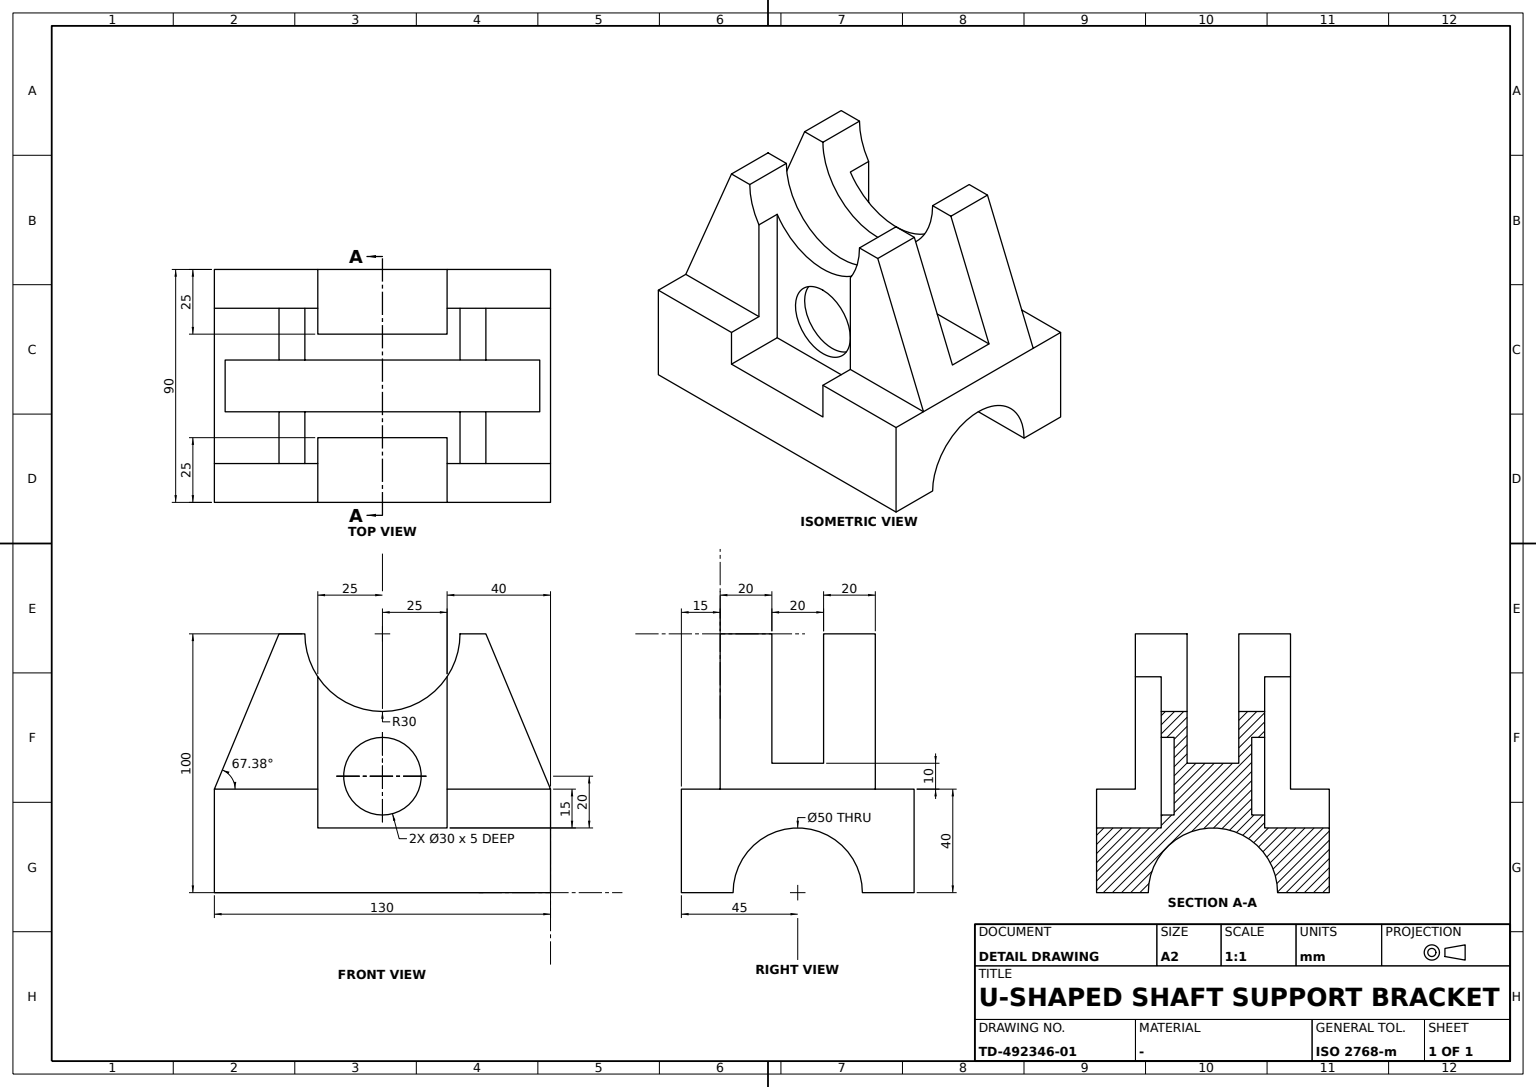
ISO-10303-21;
HEADER;
FILE_DESCRIPTION((''),'2;1');
FILE_NAME('','',(''),(''),'','','');
FILE_SCHEMA(('AUTOMOTIVE_DESIGN'));
ENDSEC;
DATA;
#1=APPLICATION_CONTEXT('');
#2=PRODUCT_CONTEXT('',#1,'mechanical');
#3=PRODUCT('','','',(#2));
#4=PRODUCT_DEFINITION_FORMATION('','',#3);
#5=PRODUCT_DEFINITION_CONTEXT('',#1,'design');
#6=PRODUCT_DEFINITION('','',#4,#5);
#7=PRODUCT_DEFINITION_SHAPE('','',#6);
#8=(LENGTH_UNIT()NAMED_UNIT(*)SI_UNIT(.MILLI.,.METRE.));
#9=(NAMED_UNIT(*)PLANE_ANGLE_UNIT()SI_UNIT($,.RADIAN.));
#10=(NAMED_UNIT(*)SI_UNIT($,.STERADIAN.)SOLID_ANGLE_UNIT());
#11=UNCERTAINTY_MEASURE_WITH_UNIT(LENGTH_MEASURE(0.005),#8,'distance_accuracy_value','');
#12=(GEOMETRIC_REPRESENTATION_CONTEXT(3)GLOBAL_UNCERTAINTY_ASSIGNED_CONTEXT((#11))GLOBAL_UNIT_ASSIGNED_CONTEXT((#8,#9,#10))REPRESENTATION_CONTEXT('',''));
#13=CARTESIAN_POINT('',(-65.,-25.,0.));
#14=VERTEX_POINT('',#13);
#15=CARTESIAN_POINT('',(65.,-25.,0.));
#16=VERTEX_POINT('',#15);
#17=DIRECTION('',(-1.,0.,0.));
#18=VECTOR('',#17,1000.);
#19=LINE('',#15,#18);
#20=EDGE_CURVE('',#14,#16,#19,.F.);
#21=ORIENTED_EDGE('',*,*,#20,.T.);
#22=CARTESIAN_POINT('',(65.,-45.,0.));
#23=VERTEX_POINT('',#22);
#24=CARTESIAN_POINT('',(65.,45.,0.));
#25=DIRECTION('',(0.,-1.,0.));
#26=VECTOR('',#25,1000.);
#27=LINE('',#24,#26);
#28=EDGE_CURVE('',#16,#23,#27,.T.);
#29=ORIENTED_EDGE('',*,*,#28,.T.);
#30=CARTESIAN_POINT('',(-65.,-45.,0.));
#31=VERTEX_POINT('',#30);
#32=LINE('',#22,#18);
#33=EDGE_CURVE('',#23,#31,#32,.T.);
#34=ORIENTED_EDGE('',*,*,#33,.T.);
#35=CARTESIAN_POINT('',(-65.,45.,0.));
#36=LINE('',#35,#26);
#37=EDGE_CURVE('',#14,#31,#36,.T.);
#38=ORIENTED_EDGE('',*,*,#37,.F.);
#39=EDGE_LOOP('',(#21,#29,#34,#38));
#40=FACE_BOUND('',#39,.T.);
#41=DIRECTION('',(0.,0.,-1.));
#42=AXIS2_PLACEMENT_3D('',#24,#41,#17);
#43=PLANE('',#42);
#44=ADVANCED_FACE('',(#40),#43,.T.);
#45=CARTESIAN_POINT('',(-25.,-30.,40.));
#46=VERTEX_POINT('',#45);
#47=CARTESIAN_POINT('',(-25.,-45.,40.));
#48=VERTEX_POINT('',#47);
#49=LINE('',#47,#26);
#50=EDGE_CURVE('',#46,#48,#49,.T.);
#51=ORIENTED_EDGE('',*,*,#50,.F.);
#52=CARTESIAN_POINT('',(-65.,-30.,40.));
#53=VERTEX_POINT('',#52);
#54=CARTESIAN_POINT('',(65.,-30.,40.));
#55=LINE('',#54,#18);
#56=EDGE_CURVE('',#46,#53,#55,.T.);
#57=ORIENTED_EDGE('',*,*,#56,.T.);
#58=CARTESIAN_POINT('',(-65.,-45.,40.));
#59=VERTEX_POINT('',#58);
#60=DIRECTION('',(0.,1.,0.));
#61=VECTOR('',#60,1000.);
#62=LINE('',#58,#61);
#63=EDGE_CURVE('',#59,#53,#62,.T.);
#64=ORIENTED_EDGE('',*,*,#63,.F.);
#65=CARTESIAN_POINT('',(65.,-45.,40.));
#66=LINE('',#65,#18);
#67=EDGE_CURVE('',#48,#59,#66,.T.);
#68=ORIENTED_EDGE('',*,*,#67,.F.);
#69=EDGE_LOOP('',(#51,#57,#64,#68));
#70=FACE_BOUND('',#69,.T.);
#71=DIRECTION('',(0.,0.,1.));
#72=DIRECTION('',(1.,0.,0.));
#73=AXIS2_PLACEMENT_3D('',#65,#71,#72);
#74=PLANE('',#73);
#75=ADVANCED_FACE('',(#70),#74,.T.);
#76=CARTESIAN_POINT('',(30.,-10.,100.));
#77=VERTEX_POINT('',#76);
#78=CARTESIAN_POINT('',(40.,-10.,100.));
#79=VERTEX_POINT('',#78);
#80=CARTESIAN_POINT('',(-40.,-10.,100.));
#81=VECTOR('',#72,1000.);
#82=LINE('',#80,#81);
#83=EDGE_CURVE('',#77,#79,#82,.T.);
#84=ORIENTED_EDGE('',*,*,#83,.F.);
#85=CARTESIAN_POINT('',(30.,-30.,100.));
#86=VERTEX_POINT('',#85);
#87=CARTESIAN_POINT('',(30.,-40.,100.));
#88=LINE('',#87,#61);
#89=EDGE_CURVE('',#77,#86,#88,.F.);
#90=ORIENTED_EDGE('',*,*,#89,.T.);
#91=CARTESIAN_POINT('',(40.,-30.,100.));
#92=VERTEX_POINT('',#91);
#93=CARTESIAN_POINT('',(-40.,-30.,100.));
#94=LINE('',#93,#81);
#95=EDGE_CURVE('',#86,#92,#94,.T.);
#96=ORIENTED_EDGE('',*,*,#95,.T.);
#97=LINE('',#91,#61);
#98=EDGE_CURVE('',#92,#79,#97,.T.);
#99=ORIENTED_EDGE('',*,*,#98,.T.);
#100=EDGE_LOOP('',(#84,#90,#96,#99));
#101=FACE_BOUND('',#100,.T.);
#102=AXIS2_PLACEMENT_3D('',#93,#71,#72);
#103=PLANE('',#102);
#104=ADVANCED_FACE('',(#101),#103,.T.);
#105=ORIENTED_EDGE('',*,*,#98,.F.);
#106=VERTEX_POINT('',#54);
#107=DIRECTION('',(0.384615385,0.,-0.923076923));
#108=VECTOR('',#107,1000.);
#109=LINE('',#91,#108);
#110=EDGE_CURVE('',#92,#106,#109,.T.);
#111=ORIENTED_EDGE('',*,*,#110,.T.);
#112=CARTESIAN_POINT('',(65.,30.,40.));
#113=VERTEX_POINT('',#112);
#114=LINE('',#54,#61);
#115=EDGE_CURVE('',#106,#113,#114,.T.);
#116=ORIENTED_EDGE('',*,*,#115,.T.);
#117=CARTESIAN_POINT('',(40.,30.,100.));
#118=VERTEX_POINT('',#117);
#119=LINE('',#117,#108);
#120=EDGE_CURVE('',#118,#113,#119,.T.);
#121=ORIENTED_EDGE('',*,*,#120,.F.);
#122=CARTESIAN_POINT('',(40.,10.,100.));
#123=VERTEX_POINT('',#122);
#124=EDGE_CURVE('',#123,#118,#97,.T.);
#125=ORIENTED_EDGE('',*,*,#124,.F.);
#126=CARTESIAN_POINT('',(60.833333,10.,50.));
#127=VERTEX_POINT('',#126);
#128=DIRECTION('',(-0.384615385,0.,0.923076923));
#129=VECTOR('',#128,1000.);
#130=LINE('',#122,#129);
#131=EDGE_CURVE('',#127,#123,#130,.T.);
#132=ORIENTED_EDGE('',*,*,#131,.F.);
#133=CARTESIAN_POINT('',(60.833333,-10.,50.));
#134=VERTEX_POINT('',#133);
#135=CARTESIAN_POINT('',(60.833333,-30.,50.));
#136=LINE('',#135,#61);
#137=EDGE_CURVE('',#134,#127,#136,.T.);
#138=ORIENTED_EDGE('',*,*,#137,.F.);
#139=LINE('',#78,#108);
#140=EDGE_CURVE('',#79,#134,#139,.T.);
#141=ORIENTED_EDGE('',*,*,#140,.F.);
#142=EDGE_LOOP('',(#105,#111,#116,#121,#125,#132,#138,#141));
#143=FACE_BOUND('',#142,.T.);
#144=DIRECTION('',(0.923076923,0.,0.384615385));
#145=AXIS2_PLACEMENT_3D('',#91,#144,#107);
#146=PLANE('',#145);
#147=ADVANCED_FACE('',(#143),#146,.T.);
#148=ORIENTED_EDGE('',*,*,#120,.T.);
#149=CARTESIAN_POINT('',(25.,30.,40.));
#150=VERTEX_POINT('',#149);
#151=LINE('',#112,#18);
#152=EDGE_CURVE('',#113,#150,#151,.T.);
#153=ORIENTED_EDGE('',*,*,#152,.T.);
#154=CARTESIAN_POINT('',(25.,30.,83.416876));
#155=VERTEX_POINT('',#154);
#156=CARTESIAN_POINT('',(25.,30.,0.));
#157=VECTOR('',#71,1000.);
#158=LINE('',#156,#157);
#159=EDGE_CURVE('',#150,#155,#158,.T.);
#160=ORIENTED_EDGE('',*,*,#159,.T.);
#161=CARTESIAN_POINT('',(30.,30.,100.));
#162=VERTEX_POINT('',#161);
#163=CARTESIAN_POINT('',(0.,30.,100.));
#164=AXIS2_PLACEMENT_3D('',#163,#60,#71);
#165=CIRCLE('',#164,30.);
#166=EDGE_CURVE('',#155,#162,#165,.F.);
#167=ORIENTED_EDGE('',*,*,#166,.T.);
#168=CARTESIAN_POINT('',(-40.,30.,100.));
#169=LINE('',#168,#81);
#170=EDGE_CURVE('',#162,#118,#169,.T.);
#171=ORIENTED_EDGE('',*,*,#170,.T.);
#172=EDGE_LOOP('',(#148,#153,#160,#167,#171));
#173=FACE_BOUND('',#172,.T.);
#174=CARTESIAN_POINT('',(0.,30.,0.));
#175=AXIS2_PLACEMENT_3D('',#174,#60,#71);
#176=PLANE('',#175);
#177=ADVANCED_FACE('',(#173),#176,.T.);
#178=CARTESIAN_POINT('',(-25.,-30.,83.416876));
#179=VERTEX_POINT('',#178);
#180=CARTESIAN_POINT('',(-25.,-20.,83.416876));
#181=VERTEX_POINT('',#180);
#182=CARTESIAN_POINT('',(-25.,-40.,83.416876));
#183=LINE('',#182,#61);
#184=EDGE_CURVE('',#179,#181,#183,.T.);
#185=ORIENTED_EDGE('',*,*,#184,.T.);
#186=CARTESIAN_POINT('',(25.,-20.,83.416876));
#187=VERTEX_POINT('',#186);
#188=CARTESIAN_POINT('',(0.,-20.,100.));
#189=AXIS2_PLACEMENT_3D('',#188,#60,#71);
#190=CIRCLE('',#189,30.);
#191=EDGE_CURVE('',#181,#187,#190,.F.);
#192=ORIENTED_EDGE('',*,*,#191,.T.);
#193=CARTESIAN_POINT('',(25.,-30.,83.416876));
#194=VERTEX_POINT('',#193);
#195=CARTESIAN_POINT('',(25.,-40.,83.416876));
#196=LINE('',#195,#61);
#197=EDGE_CURVE('',#187,#194,#196,.F.);
#198=ORIENTED_EDGE('',*,*,#197,.T.);
#199=CARTESIAN_POINT('',(0.,-30.,100.));
#200=AXIS2_PLACEMENT_3D('',#199,#60,#71);
#201=CIRCLE('',#200,30.);
#202=EDGE_CURVE('',#194,#86,#201,.F.);
#203=ORIENTED_EDGE('',*,*,#202,.T.);
#204=ORIENTED_EDGE('',*,*,#89,.F.);
#205=CARTESIAN_POINT('',(-30.,-10.,100.));
#206=VERTEX_POINT('',#205);
#207=CARTESIAN_POINT('',(0.,-10.,100.));
#208=AXIS2_PLACEMENT_3D('',#207,#25,#41);
#209=CIRCLE('',#208,30.);
#210=EDGE_CURVE('',#206,#77,#209,.T.);
#211=ORIENTED_EDGE('',*,*,#210,.F.);
#212=CARTESIAN_POINT('',(-30.,-30.,100.));
#213=VERTEX_POINT('',#212);
#214=CARTESIAN_POINT('',(-30.,-40.,100.));
#215=LINE('',#214,#61);
#216=EDGE_CURVE('',#213,#206,#215,.T.);
#217=ORIENTED_EDGE('',*,*,#216,.F.);
#218=EDGE_CURVE('',#213,#179,#201,.F.);
#219=ORIENTED_EDGE('',*,*,#218,.T.);
#220=EDGE_LOOP('',(#185,#192,#198,#203,#204,#211,#217,#219));
#221=FACE_BOUND('',#220,.T.);
#222=CARTESIAN_POINT('',(0.,-40.,100.));
#223=AXIS2_PLACEMENT_3D('',#222,#60,#71);
#224=CYLINDRICAL_SURFACE('',#223,30.);
#225=ADVANCED_FACE('',(#221),#224,.F.);
#226=CARTESIAN_POINT('',(-65.,30.,40.));
#227=VERTEX_POINT('',#226);
#228=CARTESIAN_POINT('',(-65.,45.,40.));
#229=VERTEX_POINT('',#228);
#230=EDGE_CURVE('',#227,#229,#62,.T.);
#231=ORIENTED_EDGE('',*,*,#230,.F.);
#232=CARTESIAN_POINT('',(-25.,30.,40.));
#233=VERTEX_POINT('',#232);
#234=EDGE_CURVE('',#233,#227,#151,.T.);
#235=ORIENTED_EDGE('',*,*,#234,.F.);
#236=CARTESIAN_POINT('',(-25.,45.,40.));
#237=VERTEX_POINT('',#236);
#238=LINE('',#47,#61);
#239=EDGE_CURVE('',#233,#237,#238,.T.);
#240=ORIENTED_EDGE('',*,*,#239,.T.);
#241=CARTESIAN_POINT('',(65.,45.,40.));
#242=LINE('',#241,#18);
#243=EDGE_CURVE('',#237,#229,#242,.T.);
#244=ORIENTED_EDGE('',*,*,#243,.T.);
#245=EDGE_LOOP('',(#231,#235,#240,#244));
#246=FACE_BOUND('',#245,.T.);
#247=ADVANCED_FACE('',(#246),#74,.T.);
#248=CARTESIAN_POINT('',(-60.833333,10.,50.));
#249=VERTEX_POINT('',#248);
#250=CARTESIAN_POINT('',(-70.,10.,50.));
#251=LINE('',#250,#81);
#252=EDGE_CURVE('',#127,#249,#251,.F.);
#253=ORIENTED_EDGE('',*,*,#252,.T.);
#254=CARTESIAN_POINT('',(-60.833333,-10.,50.));
#255=VERTEX_POINT('',#254);
#256=CARTESIAN_POINT('',(-60.833333,-30.,50.));
#257=LINE('',#256,#26);
#258=EDGE_CURVE('',#249,#255,#257,.T.);
#259=ORIENTED_EDGE('',*,*,#258,.T.);
#260=CARTESIAN_POINT('',(70.,-10.,50.));
#261=LINE('',#260,#18);
#262=EDGE_CURVE('',#255,#134,#261,.F.);
#263=ORIENTED_EDGE('',*,*,#262,.T.);
#264=ORIENTED_EDGE('',*,*,#137,.T.);
#265=EDGE_LOOP('',(#253,#259,#263,#264));
#266=FACE_BOUND('',#265,.T.);
#267=CARTESIAN_POINT('',(0.,0.,50.));
#268=AXIS2_PLACEMENT_3D('',#267,#41,#17);
#269=PLANE('',#268);
#270=ADVANCED_FACE('',(#266),#269,.F.);
#271=CARTESIAN_POINT('',(-30.,10.,100.));
#272=VERTEX_POINT('',#271);
#273=CARTESIAN_POINT('',(-40.,10.,100.));
#274=VERTEX_POINT('',#273);
#275=LINE('',#273,#18);
#276=EDGE_CURVE('',#272,#274,#275,.T.);
#277=ORIENTED_EDGE('',*,*,#276,.T.);
#278=CARTESIAN_POINT('',(-65.,10.,40.));
#279=DIRECTION('',(-0.384615385,0.,-0.923076923));
#280=VECTOR('',#279,1000.);
#281=LINE('',#278,#280);
#282=EDGE_CURVE('',#274,#249,#281,.T.);
#283=ORIENTED_EDGE('',*,*,#282,.T.);
#284=ORIENTED_EDGE('',*,*,#252,.F.);
#285=ORIENTED_EDGE('',*,*,#131,.T.);
#286=CARTESIAN_POINT('',(30.,10.,100.));
#287=VERTEX_POINT('',#286);
#288=EDGE_CURVE('',#123,#287,#275,.T.);
#289=ORIENTED_EDGE('',*,*,#288,.T.);
#290=CARTESIAN_POINT('',(0.,10.,100.));
#291=AXIS2_PLACEMENT_3D('',#290,#60,#71);
#292=CIRCLE('',#291,30.);
#293=EDGE_CURVE('',#287,#272,#292,.T.);
#294=ORIENTED_EDGE('',*,*,#293,.T.);
#295=EDGE_LOOP('',(#277,#283,#284,#285,#289,#294));
#296=FACE_BOUND('',#295,.T.);
#297=CARTESIAN_POINT('',(-70.,10.,104.));
#298=AXIS2_PLACEMENT_3D('',#297,#60,#71);
#299=PLANE('',#298);
#300=ADVANCED_FACE('',(#296),#299,.F.);
#301=ORIENTED_EDGE('',*,*,#202,.F.);
#302=CARTESIAN_POINT('',(25.,-30.,40.));
#303=VERTEX_POINT('',#302);
#304=CARTESIAN_POINT('',(25.,-30.,0.));
#305=VECTOR('',#41,1000.);
#306=LINE('',#304,#305);
#307=EDGE_CURVE('',#194,#303,#306,.T.);
#308=ORIENTED_EDGE('',*,*,#307,.T.);
#309=EDGE_CURVE('',#106,#303,#55,.T.);
#310=ORIENTED_EDGE('',*,*,#309,.F.);
#311=ORIENTED_EDGE('',*,*,#110,.F.);
#312=ORIENTED_EDGE('',*,*,#95,.F.);
#313=EDGE_LOOP('',(#301,#308,#310,#311,#312));
#314=FACE_BOUND('',#313,.T.);
#315=CARTESIAN_POINT('',(0.,-30.,0.));
#316=AXIS2_PLACEMENT_3D('',#315,#60,#71);
#317=PLANE('',#316);
#318=ADVANCED_FACE('',(#314),#317,.F.);
#319=VERTEX_POINT('',#24);
#320=CARTESIAN_POINT('',(65.,25.,0.));
#321=VERTEX_POINT('',#320);
#322=EDGE_CURVE('',#319,#321,#27,.T.);
#323=ORIENTED_EDGE('',*,*,#322,.F.);
#324=VERTEX_POINT('',#241);
#325=LINE('',#241,#305);
#326=EDGE_CURVE('',#324,#319,#325,.T.);
#327=ORIENTED_EDGE('',*,*,#326,.F.);
#328=LINE('',#65,#61);
#329=EDGE_CURVE('',#113,#324,#328,.T.);
#330=ORIENTED_EDGE('',*,*,#329,.F.);
#331=ORIENTED_EDGE('',*,*,#115,.F.);
#332=VERTEX_POINT('',#65);
#333=EDGE_CURVE('',#332,#106,#328,.T.);
#334=ORIENTED_EDGE('',*,*,#333,.F.);
#335=LINE('',#22,#157);
#336=EDGE_CURVE('',#23,#332,#335,.T.);
#337=ORIENTED_EDGE('',*,*,#336,.F.);
#338=ORIENTED_EDGE('',*,*,#28,.F.);
#339=CARTESIAN_POINT('',(65.,0.,0.));
#340=AXIS2_PLACEMENT_3D('',#339,#72,#60);
#341=CIRCLE('',#340,25.);
#342=EDGE_CURVE('',#321,#16,#341,.T.);
#343=ORIENTED_EDGE('',*,*,#342,.F.);
#344=EDGE_LOOP('',(#323,#327,#330,#331,#334,#337,#338,#343));
#345=FACE_BOUND('',#344,.T.);
#346=AXIS2_PLACEMENT_3D('',#339,#17,#71);
#347=PLANE('',#346);
#348=ADVANCED_FACE('',(#345),#347,.F.);
#349=CARTESIAN_POINT('',(25.,-20.,25.));
#350=VERTEX_POINT('',#349);
#351=CARTESIAN_POINT('',(25.,-20.,101.));
#352=LINE('',#351,#305);
#353=EDGE_CURVE('',#350,#187,#352,.F.);
#354=ORIENTED_EDGE('',*,*,#353,.F.);
#355=CARTESIAN_POINT('',(25.,-45.,25.));
#356=VERTEX_POINT('',#355);
#357=LINE('',#349,#26);
#358=EDGE_CURVE('',#356,#350,#357,.F.);
#359=ORIENTED_EDGE('',*,*,#358,.F.);
#360=CARTESIAN_POINT('',(25.,-45.,40.));
#361=VERTEX_POINT('',#360);
#362=CARTESIAN_POINT('',(25.,-45.,0.));
#363=LINE('',#362,#157);
#364=EDGE_CURVE('',#356,#361,#363,.T.);
#365=ORIENTED_EDGE('',*,*,#364,.T.);
#366=LINE('',#360,#61);
#367=EDGE_CURVE('',#361,#303,#366,.T.);
#368=ORIENTED_EDGE('',*,*,#367,.T.);
#369=ORIENTED_EDGE('',*,*,#307,.F.);
#370=ORIENTED_EDGE('',*,*,#197,.F.);
#371=EDGE_LOOP('',(#354,#359,#365,#368,#369,#370));
#372=FACE_BOUND('',#371,.T.);
#373=AXIS2_PLACEMENT_3D('',#351,#72,#60);
#374=PLANE('',#373);
#375=ADVANCED_FACE('',(#372),#374,.F.);
#376=VERTEX_POINT('',#93);
#377=EDGE_CURVE('',#376,#213,#94,.T.);
#378=ORIENTED_EDGE('',*,*,#377,.F.);
#379=DIRECTION('',(0.384615385,0.,0.923076923));
#380=VECTOR('',#379,1000.);
#381=LINE('',#52,#380);
#382=EDGE_CURVE('',#53,#376,#381,.T.);
#383=ORIENTED_EDGE('',*,*,#382,.F.);
#384=ORIENTED_EDGE('',*,*,#56,.F.);
#385=CARTESIAN_POINT('',(-25.,-30.,0.));
#386=LINE('',#385,#157);
#387=EDGE_CURVE('',#46,#179,#386,.T.);
#388=ORIENTED_EDGE('',*,*,#387,.T.);
#389=ORIENTED_EDGE('',*,*,#218,.F.);
#390=EDGE_LOOP('',(#378,#383,#384,#388,#389));
#391=FACE_BOUND('',#390,.T.);
#392=ADVANCED_FACE('',(#391),#317,.F.);
#393=CARTESIAN_POINT('',(25.,45.,25.));
#394=VERTEX_POINT('',#393);
#395=CARTESIAN_POINT('',(25.,20.,25.));
#396=VERTEX_POINT('',#395);
#397=LINE('',#395,#61);
#398=EDGE_CURVE('',#394,#396,#397,.F.);
#399=ORIENTED_EDGE('',*,*,#398,.T.);
#400=CARTESIAN_POINT('',(25.,20.,83.416876));
#401=VERTEX_POINT('',#400);
#402=CARTESIAN_POINT('',(25.,20.,101.));
#403=LINE('',#402,#305);
#404=EDGE_CURVE('',#396,#401,#403,.F.);
#405=ORIENTED_EDGE('',*,*,#404,.T.);
#406=EDGE_CURVE('',#401,#155,#196,.T.);
#407=ORIENTED_EDGE('',*,*,#406,.T.);
#408=ORIENTED_EDGE('',*,*,#159,.F.);
#409=CARTESIAN_POINT('',(25.,45.,40.));
#410=VERTEX_POINT('',#409);
#411=LINE('',#360,#26);
#412=EDGE_CURVE('',#410,#150,#411,.T.);
#413=ORIENTED_EDGE('',*,*,#412,.F.);
#414=LINE('',#409,#157);
#415=EDGE_CURVE('',#394,#410,#414,.T.);
#416=ORIENTED_EDGE('',*,*,#415,.F.);
#417=EDGE_LOOP('',(#399,#405,#407,#408,#413,#416));
#418=FACE_BOUND('',#417,.T.);
#419=AXIS2_PLACEMENT_3D('',#402,#17,#25);
#420=PLANE('',#419);
#421=ADVANCED_FACE('',(#418),#420,.T.);
#422=CARTESIAN_POINT('',(-65.,25.,0.));
#423=VERTEX_POINT('',#422);
#424=LINE('',#320,#18);
#425=EDGE_CURVE('',#321,#423,#424,.T.);
#426=ORIENTED_EDGE('',*,*,#425,.T.);
#427=VERTEX_POINT('',#35);
#428=EDGE_CURVE('',#427,#423,#36,.T.);
#429=ORIENTED_EDGE('',*,*,#428,.F.);
#430=LINE('',#24,#18);
#431=EDGE_CURVE('',#319,#427,#430,.T.);
#432=ORIENTED_EDGE('',*,*,#431,.F.);
#433=ORIENTED_EDGE('',*,*,#322,.T.);
#434=EDGE_LOOP('',(#426,#429,#432,#433));
#435=FACE_BOUND('',#434,.T.);
#436=ADVANCED_FACE('',(#435),#43,.T.);
#437=ORIENTED_EDGE('',*,*,#152,.F.);
#438=ORIENTED_EDGE('',*,*,#329,.T.);
#439=EDGE_CURVE('',#324,#410,#242,.T.);
#440=ORIENTED_EDGE('',*,*,#439,.T.);
#441=ORIENTED_EDGE('',*,*,#412,.T.);
#442=EDGE_LOOP('',(#437,#438,#440,#441));
#443=FACE_BOUND('',#442,.T.);
#444=ADVANCED_FACE('',(#443),#74,.T.);
#445=ORIENTED_EDGE('',*,*,#398,.F.);
#446=CARTESIAN_POINT('',(-25.,45.,25.));
#447=VERTEX_POINT('',#446);
#448=CARTESIAN_POINT('',(65.,45.,25.));
#449=LINE('',#448,#81);
#450=EDGE_CURVE('',#447,#394,#449,.T.);
#451=ORIENTED_EDGE('',*,*,#450,.F.);
#452=CARTESIAN_POINT('',(-25.,20.,25.));
#453=VERTEX_POINT('',#452);
#454=CARTESIAN_POINT('',(-25.,54.,25.));
#455=LINE('',#454,#26);
#456=EDGE_CURVE('',#453,#447,#455,.F.);
#457=ORIENTED_EDGE('',*,*,#456,.F.);
#458=LINE('',#452,#81);
#459=EDGE_CURVE('',#396,#453,#458,.F.);
#460=ORIENTED_EDGE('',*,*,#459,.F.);
#461=EDGE_LOOP('',(#445,#451,#457,#460));
#462=FACE_BOUND('',#461,.T.);
#463=CARTESIAN_POINT('',(0.,0.,25.));
#464=AXIS2_PLACEMENT_3D('',#463,#71,#72);
#465=PLANE('',#464);
#466=ADVANCED_FACE('',(#462),#465,.T.);
#467=CARTESIAN_POINT('',(0.,15.,30.));
#468=VERTEX_POINT('',#467);
#469=CARTESIAN_POINT('',(0.,15.,45.));
#470=AXIS2_PLACEMENT_3D('',#469,#25,#41);
#471=CIRCLE('',#470,15.);
#472=EDGE_CURVE('',#468,#468,#471,.T.);
#473=ORIENTED_EDGE('',*,*,#472,.T.);
#474=EDGE_LOOP('',(#473));
#475=FACE_BOUND('',#474,.T.);
#476=CARTESIAN_POINT('',(0.,20.,30.));
#477=VERTEX_POINT('',#476);
#478=CARTESIAN_POINT('',(0.,20.,45.));
#479=AXIS2_PLACEMENT_3D('',#478,#25,#41);
#480=CIRCLE('',#479,15.);
#481=EDGE_CURVE('',#477,#477,#480,.T.);
#482=ORIENTED_EDGE('',*,*,#481,.F.);
#483=EDGE_LOOP('',(#482));
#484=FACE_BOUND('',#483,.T.);
#485=CYLINDRICAL_SURFACE('',#479,15.);
#486=ADVANCED_FACE('',(#475,#484),#485,.F.);
#487=ORIENTED_EDGE('',*,*,#481,.T.);
#488=EDGE_LOOP('',(#487));
#489=FACE_BOUND('',#488,.T.);
#490=ORIENTED_EDGE('',*,*,#404,.F.);
#491=ORIENTED_EDGE('',*,*,#459,.T.);
#492=CARTESIAN_POINT('',(-25.,20.,83.416876));
#493=VERTEX_POINT('',#492);
#494=CARTESIAN_POINT('',(-25.,20.,101.));
#495=LINE('',#494,#305);
#496=EDGE_CURVE('',#453,#493,#495,.F.);
#497=ORIENTED_EDGE('',*,*,#496,.T.);
#498=CARTESIAN_POINT('',(0.,20.,100.));
#499=AXIS2_PLACEMENT_3D('',#498,#60,#71);
#500=CIRCLE('',#499,30.);
#501=EDGE_CURVE('',#493,#401,#500,.F.);
#502=ORIENTED_EDGE('',*,*,#501,.T.);
#503=EDGE_LOOP('',(#490,#491,#497,#502));
#504=FACE_BOUND('',#503,.T.);
#505=AXIS2_PLACEMENT_3D('',#494,#60,#71);
#506=PLANE('',#505);
#507=ADVANCED_FACE('',(#489,#504),#506,.T.);
#508=VERTEX_POINT('',#168);
#509=CARTESIAN_POINT('',(-30.,30.,100.));
#510=VERTEX_POINT('',#509);
#511=EDGE_CURVE('',#508,#510,#169,.T.);
#512=ORIENTED_EDGE('',*,*,#511,.F.);
#513=LINE('',#93,#61);
#514=EDGE_CURVE('',#274,#508,#513,.T.);
#515=ORIENTED_EDGE('',*,*,#514,.F.);
#516=ORIENTED_EDGE('',*,*,#276,.F.);
#517=EDGE_CURVE('',#272,#510,#215,.T.);
#518=ORIENTED_EDGE('',*,*,#517,.T.);
#519=EDGE_LOOP('',(#512,#515,#516,#518));
#520=FACE_BOUND('',#519,.T.);
#521=ADVANCED_FACE('',(#520),#103,.T.);
#522=ORIENTED_EDGE('',*,*,#216,.T.);
#523=VERTEX_POINT('',#80);
#524=EDGE_CURVE('',#523,#206,#82,.T.);
#525=ORIENTED_EDGE('',*,*,#524,.F.);
#526=EDGE_CURVE('',#376,#523,#513,.T.);
#527=ORIENTED_EDGE('',*,*,#526,.F.);
#528=ORIENTED_EDGE('',*,*,#377,.T.);
#529=EDGE_LOOP('',(#522,#525,#527,#528));
#530=FACE_BOUND('',#529,.T.);
#531=ADVANCED_FACE('',(#530),#103,.T.);
#532=ORIENTED_EDGE('',*,*,#184,.F.);
#533=ORIENTED_EDGE('',*,*,#387,.F.);
#534=ORIENTED_EDGE('',*,*,#50,.T.);
#535=CARTESIAN_POINT('',(-25.,-45.,25.));
#536=VERTEX_POINT('',#535);
#537=CARTESIAN_POINT('',(-25.,-45.,0.));
#538=LINE('',#537,#305);
#539=EDGE_CURVE('',#48,#536,#538,.T.);
#540=ORIENTED_EDGE('',*,*,#539,.T.);
#541=CARTESIAN_POINT('',(-25.,-20.,25.));
#542=VERTEX_POINT('',#541);
#543=CARTESIAN_POINT('',(-25.,-54.,25.));
#544=LINE('',#543,#61);
#545=EDGE_CURVE('',#542,#536,#544,.F.);
#546=ORIENTED_EDGE('',*,*,#545,.F.);
#547=CARTESIAN_POINT('',(-25.,-20.,101.));
#548=LINE('',#547,#305);
#549=EDGE_CURVE('',#542,#181,#548,.F.);
#550=ORIENTED_EDGE('',*,*,#549,.T.);
#551=EDGE_LOOP('',(#532,#533,#534,#540,#546,#550));
#552=FACE_BOUND('',#551,.T.);
#553=CARTESIAN_POINT('',(-25.,-54.,101.));
#554=AXIS2_PLACEMENT_3D('',#553,#17,#25);
#555=PLANE('',#554);
#556=ADVANCED_FACE('',(#552),#555,.F.);
#557=ORIENTED_EDGE('',*,*,#431,.T.);
#558=LINE('',#228,#305);
#559=EDGE_CURVE('',#229,#427,#558,.T.);
#560=ORIENTED_EDGE('',*,*,#559,.F.);
#561=ORIENTED_EDGE('',*,*,#243,.F.);
#562=LINE('',#236,#305);
#563=EDGE_CURVE('',#237,#447,#562,.T.);
#564=ORIENTED_EDGE('',*,*,#563,.T.);
#565=ORIENTED_EDGE('',*,*,#450,.T.);
#566=ORIENTED_EDGE('',*,*,#415,.T.);
#567=ORIENTED_EDGE('',*,*,#439,.F.);
#568=ORIENTED_EDGE('',*,*,#326,.T.);
#569=EDGE_LOOP('',(#557,#560,#561,#564,#565,#566,#567,#568));
#570=FACE_BOUND('',#569,.T.);
#571=AXIS2_PLACEMENT_3D('',#241,#60,#71);
#572=PLANE('',#571);
#573=ADVANCED_FACE('',(#570),#572,.T.);
#574=ORIENTED_EDGE('',*,*,#333,.T.);
#575=ORIENTED_EDGE('',*,*,#309,.T.);
#576=ORIENTED_EDGE('',*,*,#367,.F.);
#577=EDGE_CURVE('',#332,#361,#66,.T.);
#578=ORIENTED_EDGE('',*,*,#577,.F.);
#579=EDGE_LOOP('',(#574,#575,#576,#578));
#580=FACE_BOUND('',#579,.T.);
#581=ADVANCED_FACE('',(#580),#74,.T.);
#582=LINE('',#541,#81);
#583=EDGE_CURVE('',#350,#542,#582,.F.);
#584=ORIENTED_EDGE('',*,*,#583,.F.);
#585=ORIENTED_EDGE('',*,*,#353,.T.);
#586=ORIENTED_EDGE('',*,*,#191,.F.);
#587=ORIENTED_EDGE('',*,*,#549,.F.);
#588=EDGE_LOOP('',(#584,#585,#586,#587));
#589=FACE_BOUND('',#588,.T.);
#590=CARTESIAN_POINT('',(0.,-20.,60.));
#591=VERTEX_POINT('',#590);
#592=CARTESIAN_POINT('',(0.,-20.,45.));
#593=AXIS2_PLACEMENT_3D('',#592,#60,#71);
#594=CIRCLE('',#593,15.);
#595=EDGE_CURVE('',#591,#591,#594,.T.);
#596=ORIENTED_EDGE('',*,*,#595,.T.);
#597=EDGE_LOOP('',(#596));
#598=FACE_BOUND('',#597,.T.);
#599=AXIS2_PLACEMENT_3D('',#547,#60,#71);
#600=PLANE('',#599);
#601=ADVANCED_FACE('',(#589,#598),#600,.F.);
#602=EDGE_CURVE('',#162,#287,#88,.F.);
#603=ORIENTED_EDGE('',*,*,#602,.T.);
#604=ORIENTED_EDGE('',*,*,#288,.F.);
#605=ORIENTED_EDGE('',*,*,#124,.T.);
#606=ORIENTED_EDGE('',*,*,#170,.F.);
#607=EDGE_LOOP('',(#603,#604,#605,#606));
#608=FACE_BOUND('',#607,.T.);
#609=ADVANCED_FACE('',(#608),#103,.T.);
#610=ORIENTED_EDGE('',*,*,#496,.F.);
#611=ORIENTED_EDGE('',*,*,#456,.T.);
#612=ORIENTED_EDGE('',*,*,#563,.F.);
#613=ORIENTED_EDGE('',*,*,#239,.F.);
#614=CARTESIAN_POINT('',(-25.,30.,83.416876));
#615=VERTEX_POINT('',#614);
#616=CARTESIAN_POINT('',(-25.,30.,0.));
#617=LINE('',#616,#305);
#618=EDGE_CURVE('',#615,#233,#617,.T.);
#619=ORIENTED_EDGE('',*,*,#618,.F.);
#620=EDGE_CURVE('',#615,#493,#183,.F.);
#621=ORIENTED_EDGE('',*,*,#620,.T.);
#622=EDGE_LOOP('',(#610,#611,#612,#613,#619,#621));
#623=FACE_BOUND('',#622,.T.);
#624=CARTESIAN_POINT('',(-25.,54.,101.));
#625=AXIS2_PLACEMENT_3D('',#624,#72,#60);
#626=PLANE('',#625);
#627=ADVANCED_FACE('',(#623),#626,.T.);
#628=CARTESIAN_POINT('',(0.,-15.,60.));
#629=VERTEX_POINT('',#628);
#630=CARTESIAN_POINT('',(0.,-15.,45.));
#631=AXIS2_PLACEMENT_3D('',#630,#60,#71);
#632=CIRCLE('',#631,15.);
#633=EDGE_CURVE('',#629,#629,#632,.F.);
#634=ORIENTED_EDGE('',*,*,#633,.F.);
#635=EDGE_LOOP('',(#634));
#636=FACE_BOUND('',#635,.T.);
#637=ORIENTED_EDGE('',*,*,#595,.F.);
#638=EDGE_LOOP('',(#637));
#639=FACE_BOUND('',#638,.T.);
#640=CYLINDRICAL_SURFACE('',#593,15.);
#641=ADVANCED_FACE('',(#636,#639),#640,.F.);
#642=ORIENTED_EDGE('',*,*,#262,.F.);
#643=CARTESIAN_POINT('',(-65.,-10.,40.));
#644=LINE('',#643,#380);
#645=EDGE_CURVE('',#255,#523,#644,.T.);
#646=ORIENTED_EDGE('',*,*,#645,.T.);
#647=ORIENTED_EDGE('',*,*,#524,.T.);
#648=ORIENTED_EDGE('',*,*,#210,.T.);
#649=ORIENTED_EDGE('',*,*,#83,.T.);
#650=ORIENTED_EDGE('',*,*,#140,.T.);
#651=EDGE_LOOP('',(#642,#646,#647,#648,#649,#650));
#652=FACE_BOUND('',#651,.T.);
#653=CARTESIAN_POINT('',(70.,-10.,104.));
#654=AXIS2_PLACEMENT_3D('',#653,#25,#41);
#655=PLANE('',#654);
#656=ADVANCED_FACE('',(#652),#655,.F.);
#657=ORIENTED_EDGE('',*,*,#358,.T.);
#658=ORIENTED_EDGE('',*,*,#583,.T.);
#659=ORIENTED_EDGE('',*,*,#545,.T.);
#660=CARTESIAN_POINT('',(65.,-45.,25.));
#661=LINE('',#660,#81);
#662=EDGE_CURVE('',#536,#356,#661,.T.);
#663=ORIENTED_EDGE('',*,*,#662,.T.);
#664=EDGE_LOOP('',(#657,#658,#659,#663));
#665=FACE_BOUND('',#664,.T.);
#666=AXIS2_PLACEMENT_3D('',#463,#41,#17);
#667=PLANE('',#666);
#668=ADVANCED_FACE('',(#665),#667,.F.);
#669=ORIENTED_EDGE('',*,*,#293,.F.);
#670=ORIENTED_EDGE('',*,*,#602,.F.);
#671=ORIENTED_EDGE('',*,*,#166,.F.);
#672=ORIENTED_EDGE('',*,*,#406,.F.);
#673=ORIENTED_EDGE('',*,*,#501,.F.);
#674=ORIENTED_EDGE('',*,*,#620,.F.);
#675=EDGE_CURVE('',#510,#615,#165,.F.);
#676=ORIENTED_EDGE('',*,*,#675,.F.);
#677=ORIENTED_EDGE('',*,*,#517,.F.);
#678=EDGE_LOOP('',(#669,#670,#671,#672,#673,#674,#676,#677));
#679=FACE_BOUND('',#678,.T.);
#680=ADVANCED_FACE('',(#679),#224,.F.);
#681=ORIENTED_EDGE('',*,*,#33,.F.);
#682=ORIENTED_EDGE('',*,*,#336,.T.);
#683=ORIENTED_EDGE('',*,*,#577,.T.);
#684=ORIENTED_EDGE('',*,*,#364,.F.);
#685=ORIENTED_EDGE('',*,*,#662,.F.);
#686=ORIENTED_EDGE('',*,*,#539,.F.);
#687=ORIENTED_EDGE('',*,*,#67,.T.);
#688=LINE('',#30,#157);
#689=EDGE_CURVE('',#31,#59,#688,.T.);
#690=ORIENTED_EDGE('',*,*,#689,.F.);
#691=EDGE_LOOP('',(#681,#682,#683,#684,#685,#686,#687,#690));
#692=FACE_BOUND('',#691,.T.);
#693=AXIS2_PLACEMENT_3D('',#22,#25,#41);
#694=PLANE('',#693);
#695=ADVANCED_FACE('',(#692),#694,.T.);
#696=ORIENTED_EDGE('',*,*,#633,.T.);
#697=EDGE_LOOP('',(#696));
#698=FACE_BOUND('',#697,.T.);
#699=PLANE('',#631);
#700=ADVANCED_FACE('',(#698),#699,.F.);
#701=ORIENTED_EDGE('',*,*,#234,.T.);
#702=LINE('',#226,#380);
#703=EDGE_CURVE('',#227,#508,#702,.T.);
#704=ORIENTED_EDGE('',*,*,#703,.T.);
#705=ORIENTED_EDGE('',*,*,#511,.T.);
#706=ORIENTED_EDGE('',*,*,#675,.T.);
#707=ORIENTED_EDGE('',*,*,#618,.T.);
#708=EDGE_LOOP('',(#701,#704,#705,#706,#707));
#709=FACE_BOUND('',#708,.T.);
#710=ADVANCED_FACE('',(#709),#176,.T.);
#711=ORIENTED_EDGE('',*,*,#472,.F.);
#712=EDGE_LOOP('',(#711));
#713=FACE_BOUND('',#712,.T.);
#714=PLANE('',#470);
#715=ADVANCED_FACE('',(#713),#714,.F.);
#716=ORIENTED_EDGE('',*,*,#425,.F.);
#717=ORIENTED_EDGE('',*,*,#342,.T.);
#718=ORIENTED_EDGE('',*,*,#20,.F.);
#719=CARTESIAN_POINT('',(-65.,0.,0.));
#720=AXIS2_PLACEMENT_3D('',#719,#17,#71);
#721=CIRCLE('',#720,25.);
#722=EDGE_CURVE('',#423,#14,#721,.F.);
#723=ORIENTED_EDGE('',*,*,#722,.F.);
#724=EDGE_LOOP('',(#716,#717,#718,#723));
#725=FACE_BOUND('',#724,.T.);
#726=CYLINDRICAL_SURFACE('',#346,25.);
#727=ADVANCED_FACE('',(#725),#726,.F.);
#728=ORIENTED_EDGE('',*,*,#703,.F.);
#729=LINE('',#52,#61);
#730=EDGE_CURVE('',#53,#227,#729,.T.);
#731=ORIENTED_EDGE('',*,*,#730,.F.);
#732=ORIENTED_EDGE('',*,*,#382,.T.);
#733=ORIENTED_EDGE('',*,*,#526,.T.);
#734=ORIENTED_EDGE('',*,*,#645,.F.);
#735=ORIENTED_EDGE('',*,*,#258,.F.);
#736=ORIENTED_EDGE('',*,*,#282,.F.);
#737=ORIENTED_EDGE('',*,*,#514,.T.);
#738=EDGE_LOOP('',(#728,#731,#732,#733,#734,#735,#736,#737));
#739=FACE_BOUND('',#738,.T.);
#740=DIRECTION('',(-0.923076923,0.,0.384615385));
#741=AXIS2_PLACEMENT_3D('',#52,#740,#379);
#742=PLANE('',#741);
#743=ADVANCED_FACE('',(#739),#742,.T.);
#744=ORIENTED_EDGE('',*,*,#559,.T.);
#745=ORIENTED_EDGE('',*,*,#428,.T.);
#746=ORIENTED_EDGE('',*,*,#722,.T.);
#747=ORIENTED_EDGE('',*,*,#37,.T.);
#748=ORIENTED_EDGE('',*,*,#689,.T.);
#749=ORIENTED_EDGE('',*,*,#63,.T.);
#750=ORIENTED_EDGE('',*,*,#730,.T.);
#751=ORIENTED_EDGE('',*,*,#230,.T.);
#752=EDGE_LOOP('',(#744,#745,#746,#747,#748,#749,#750,#751));
#753=FACE_BOUND('',#752,.T.);
#754=PLANE('',#720);
#755=ADVANCED_FACE('',(#753),#754,.T.);
#756=CLOSED_SHELL('',(#44,#75,#104,#147,#177,#225,#247,#270,#300,#318,#348,#375,#392,#421,#436,#444,#466,#486,#507,#521,#531,#556,#573,#581,#601,#609,#627,#641,#656,#668,#680,#695,#700,#710,#715,#727,#743,#755));
#757=MANIFOLD_SOLID_BREP('',#756);
#758=ADVANCED_BREP_SHAPE_REPRESENTATION('',(#757),#12);
#759=SHAPE_DEFINITION_REPRESENTATION(#7,#758);
ENDSEC;
END-ISO-10303-21;
